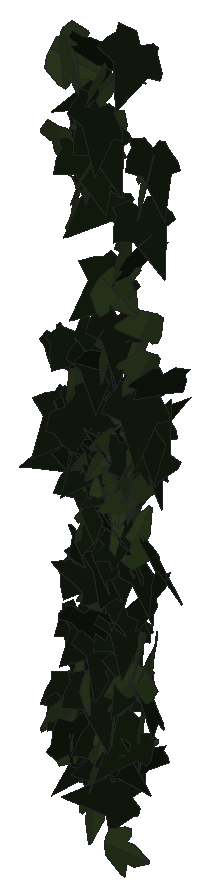
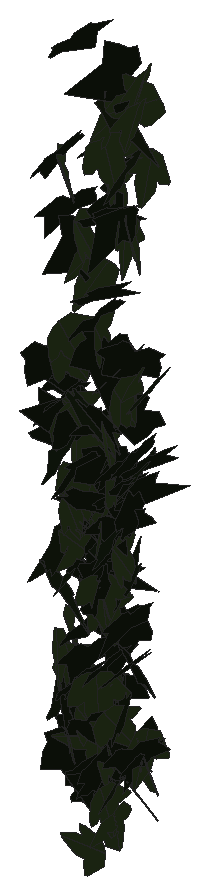
# SketchUp Ruby script. Lengths in inches.
U = 1.inch
M = Sketchup.active_model
def pt(a) = Geom::Point3d.new(a.map { |v| v * U })
def face(e, loops, mat)
  f = e.add_face(loops[0].map { |a| pt(a) })
  loops[1..].each { |l| e.add_face(l.map { |a| pt(a) }).erase! }
  f.material = f.back_material = mat if mat
  f
end
# faces: each face lists its corners as indices into pts; further lists are holes
def faces(e, pts, list, mat = nil) = list.each { |f| face(e, (f[0].is_a?(Array) ? f : [f]).map { |l| l.map { |i| pts[i] } }, mat) }
# xy, xz, yz: faces in a plane at the given z, y or x. An outline is a flat list of corners, or four numbers for a rectangle; further outlines are holes
def ring(l) = l.size == 4 ? [[l[0], l[1]], [l[2], l[1]], [l[2], l[3]], [l[0], l[3]]] : l.each_slice(2).to_a
def flat(e, list, mat, &to3) = list.each { |f| face(e, (f[0].is_a?(Array) ? f : [f]).map { |l| ring(l).map { |u, v| to3.(u, v) } }, mat) }
def xy(e, z, list, mat = nil) = flat(e, list, mat) { |x, y| [x, y, z] }
def xz(e, y, list, mat = nil) = flat(e, list, mat) { |x, z| [x, y, z] }
def yz(e, x, list, mat = nil) = flat(e, list, mat) { |y, z| [x, y, z] }
def lines(e, pts, list) = list.each { |a, b| e.add_line(pt(pts[a]), pt(pts[b])) }
# prism: a flat outline (further loops are holes) pulled along v
def prism(e, loops, v, mat = nil)
  f = face(e, loops, mat); d = Geom::Vector3d.new(v.map { |x| x * U })
  f.pushpull(f.normal.samedirection?(d) ? d.length : -d.length)
end
def box(e, o, s, mat = nil) = prism(e, [[o, [o[0] + s[0], o[1], o[2]], [o[0] + s[0], o[1] + s[1], o[2]], [o[0], o[1] + s[1], o[2]]]], [0, 0, s[2]], mat)
def at(x, y, z, deg = 0) = Geom::Transformation.translation(pt([x, y, z])) * Geom::Transformation.rotation(ORIGIN, Z_AXIS, deg.degrees)
def axes(o, x, y, z) = Geom::Transformation.new([*x, 0, *y, 0, *z, 0, *pt(o).to_a, 1])
def part(name) = M.definitions.add(name)
# library, detail: a bought-in or finely detailed component or shape, given as its bounding box
def library(name, o, s) = part(name).tap { |d| box(d.entities, o, s) }
def detail(e, o, s) = box(e.add_group.entities, o, s)
def put(e, d, t, mat = nil) = e.add_instance(d, t).tap { |i| i.material = mat if mat }
def group(e, t, mat = nil) = e.add_group.tap { |g| g.transformation = t; g.material = mat if mat }.entities
root = M.entities
M.materials.add("efeu1").color = [18, 25, 13]
M.materials.add("efeu2").color = [43, 57, 29]
c1 = part("ivyleaf_9")
p = [[1.54,2.16,1.25],[1.36,2.04,1.19],[-0.21,0.99,0.68],[-0.71,1.11,0.82],[-0.85,0.86,0.67],[-0.8,0.17,0.21],
  [-0.9,-0.01,0.1],[-0.67,-0.16,-0.02],[-0.08,-0.08,-0.05],[-0.03,-0.6,-0.4],[0.65,-0.88,-0.66],[0.83,-0.6,-0.49],
  [1.29,-0.42,-0.43],[1.8125,-0.07,-0.26],[1.21,0.44,0.15]]
faces(c1.entities,p,[[0,1,2,3,4,5,6,7,8,9,10,11,12,13,14]],"efeu1")
c2 = part("ivyleaf_10")
p = [[0,0.5,-0.03],[-0.0625,2.02,-0.43],[-0.19,2.01,-0.46],[-0.54,1.05,-0.29],[-0.52,0.625,-0.18],[-0.83,0.76,-0.28],
  [-1.16,0.64,-0.33],[-1.15,0.33,-0.24],[-0.77,-0.39,0.02],[-0.3,-0.51,0.16],[0.04,-0.48,0.23],[-0.02,2.01,-0.4375],
  [-0.06,2.01,-0.43],[0.04,-0.49,0.23],[0.67,-0.49,0.14],[1.38,0.36,-0.2],[1.375,0.51,-0.24],[0.81,0.65,-0.19],
  [0.62,0.59,-0.15],[0.6,1.09,-0.28],[0.5,1.23,-0.31]]
faces(c2.entities,p,[[0,1,2,3,4,5,6,7,8,9,10],[11,12,0,13,14,15,16,17,18,19,20]],"efeu2")
put(root,c1,axes([547.32,131.42,224.66],[-0.47868,-0.70634,0.46293],[-0.07674,-0.49354,-0.8324],[0.84104,-0.44705,0.18753]))
put(root,c1,axes([547.71,131.58,223.14],[-0.49322,-0.36938,0.71696],[-0.52746,-0.48802,-0.61429],[0.61013,-0.7205,0.04852]))
put(root,c1,axes([547.15,132.01,211.76],[-0.22016,-0.88269,-0.2571],[0.05857,0.25037,-0.90972],[0.9175,-0.22779,-0.00362]))
put(root,c1,axes([547.45,132.16,222.26],[-0.04191,-0.03531,0.93001],[-0.38732,-0.84584,-0.04957],[0.84625,-0.38888,0.02337]))
put(root,c2,axes([547.47,130.75,211.55],[-0.18429,-0.84828,-0.40002],[0.1268,0.38139,-0.86719],[0.92926,-0.22027,0.039]))
put(root,c1,axes([547.14,131.29,211.23],[0.26036,-0.7735,-0.32739],[-0.09812,0.3124,-0.81612],[0.83418,0.27816,0.00618]))
put(root,c1,axes([547.01,130.96,228.1875],[0.58686,-0.6803,-0.30129],[-0.06346,0.33656,-0.88357],[0.74132,0.56737,0.16287]))
put(root,c2,axes([547.39,131.55,241.125],[-0.02007,0.99355,0.08252],[0.00579,0.08265,-0.99372],[-0.99695,-0.01953,-0.00743]))
put(root,c2,axes([547.71,130.32,238.18],[-0.98634,0.09088,0.02629],[-0.02805,-0.01793,-0.99031],[-0.09035,-0.98653,0.02042]))
put(root,c2,axes([547.59,130.89,242.27],[-0.23804,0.98869,0.08205],[-0.01701,0.0803,-1.01694],[-0.99194,-0.23864,-0.00225]))
put(root,c2,axes([547.66,131.57,235.55],[0.54123,-0.82841,0.07096],[0.05419,-0.04934,-0.98937],[0.82967,0.54362,0.01833]))
put(root,c2,axes([547.33,130.66,209.71],[0.83861,-0.57924,-0.33432],[0.2838,-0.17731,1.0191],[-0.6056,-0.88521,0.01463]))
put(root,c1,axes([547.26,131.54,224.36],[0.3636,-0.84522,0.18301],[0.08963,-0.16063,-0.91993],[0.86015,0.37403,0.01849]))
put(root,c1,axes([547.47,131.55,215.46],[-0.46735,-0.24401,-0.71496],[0.74885,-0.03877,-0.47627],[0.09963,-0.85327,0.2261]))
put(root,c2,axes([547.24,130.92,241.41],[0.31548,0.25093,0.93435],[0.69363,0.62644,-0.40243],[-0.67443,0.76165,0.02317]))
put(root,c1,axes([547.54,131.38,225.12],[0.34402,-0.81704,-0.3168],[-0.126,0.29068,-0.88651],[0.8672,0.36636,-0.00313]))
put(root,c1,axes([547.64,131.59,217.67],[0.26274,-0.70515,-0.50734],[-0.07363,0.51005,-0.74705],[0.86557,0.25744,0.09045]))
put(root,c2,axes([547.63,131.04,210.85],[-0.20357,0.20119,-0.88456],[0.38608,-0.80114,-0.27107],[-0.82089,-0.42668,0.09188]))
put(root,c1,axes([547.73,132.27,212.72],[-0.0895,-0.19387,0.91513],[0.13572,-0.91228,-0.17999],[0.92554,0.11503,0.11488]))
put(root,c2,axes([548.24,132.12,212.84],[-0.40315,-0.58171,0.56523],[-0.04105,-0.61576,-0.663],[0.81006,-0.32072,0.24771]))
put(root,c2,axes([548.1,131.71,220.34],[0.27034,-0.74396,0.51626],[0.19524,-0.47821,-0.79138],[0.88424,0.33304,0.0169]))
put(root,c2,axes([548.3,131.02,235.13],[0.15158,-0.92217,-0.3501],[0.02552,0.35776,-0.93129],[0.98606,0.1325,0.07792]))
put(root,c1,axes([548.25,131.75,214.76],[-0.39192,-0.63578,0.60141],[-0.03798,-0.64598,-0.70765],[0.87433,-0.31305,0.23884]))
put(root,c1,axes([547.9,131.8,224.8],[0.28671,-0.85198,-0.28202],[0.00517,0.29762,-0.89387],[0.89743,0.27047,0.09525]))
put(root,c1,axes([548.9375,131.03,240.46],[-0.70581,0.71174,-0.00258],[-0.13908,-0.14148,-0.98254],[-0.69802,-0.69149,0.19838]))
put(root,c1,axes([548.15,131.79,222.04],[-0.3064,-0.87543,-0.31963],[0.13386,0.29163,-0.92707],[0.92229,-0.33316,0.02837]))
put(root,c2,axes([548.06,131.22,227.31],[-0.09751,-0.30544,0.97975],[0.5556,-0.84317,-0.20756],[0.86285,0.50841,0.24437]))
put(root,c1,axes([548.78,130.81,209.66],[-0.83384,0.27462,-0.12822],[0.11727,-0.05375,-0.87778],[-0.27947,-0.84193,0.01421]))
put(root,c1,axes([548.29,131.38,236.13],[0.91272,0.16773,-0.33496],[-0.34294,0.0191,-0.92489],[-0.15075,0.97206,0.07597]))
put(root,c1,axes([548.47,131.75,223.1],[-0.42551,-0.70439,0.44819],[-0.11444,-0.44909,-0.81444],[0.82701,-0.42456,0.1179]))
put(root,c1,axes([548.12,131.4,218.51],[0.62788,-0.5745,-0.46011],[0.38815,-0.25542,0.84858],[-0.62538,-0.73532,0.06473]))
put(root,c2,axes([548.41,131.29,227.4],[0.11453,-0.81074,0.55762],[0.24872,-0.5193,-0.80612],[0.95204,0.2332,0.14352]))
put(root,c1,axes([547.98,131.49,238],[0.5069,-0.83393,0.20261],[0.10523,-0.17314,-0.9759],[0.85171,0.51771,-0.00002]))
put(root,c2,axes([548.64,131.25,223.44],[0.07915,-0.92586,0.10516],[0.02453,-0.10343,-0.92911],[0.93149,0.0814,0.01553]))
put(root,c1,axes([548.45,129.94,210.08],[-0.17006,-0.19771,0.96973],[0.68393,0.68771,0.26015],[-0.71533,0.70452,0.0182]))
put(root,c1,axes([548.15,132.06,221.29],[0.52736,-0.78971,0.23886],[0.10385,-0.21769,-0.94901],[0.81848,0.53644,-0.03348]))
put(root,c2,axes([549.01,130.94,240.05],[0.01364,-0.0121,1.00923],[-0.41848,0.9184,0.01667],[-0.91845,-0.41864,0.00739]))
put(root,c2,axes([549.04,131.82,218.66],[-0.78887,-0.39575,0.18638],[-0.1283,-0.15811,-0.87876],[0.4182,-0.79502,0.08199]))
put(root,c1,axes([548.38,130.44,229.11],[-0.10535,-0.57039,-0.78902],[0.32065,0.72902,-0.56983],[0.91928,-0.31965,0.10833]))
put(root,c2,axes([548.9375,131.49,225.71],[0.37454,-0.85823,-0.17643],[-0.05543,0.16828,-0.93626],[0.87442,0.37828,0.01622]))
put(root,c1,axes([548.57,131.3125,223.78],[0.62831,-0.58568,-0.45673],[-0.32691,0.31909,-0.8589],[0.6669,0.7082,0.00927]))
put(root,c2,axes([549.03,131.46,238.83],[-0.48059,-0.84701,0.21226],[-0.02972,-0.22628,-0.97024],[0.87269,-0.47415,0.08385]))
put(root,c2,axes([548.78,131.22,207.66],[0.09175,0.92056,-0.34703],[-0.05828,-0.34284,-0.92485],[-0.98207,0.10635,0.02246]))
put(root,c1,axes([549.3,131.29,218.85],[-0.76483,-0.53418,0.18892],[0.16843,0.08868,0.93262],[-0.54099,0.78281,0.02326]))
put(root,c2,axes([548.99,131.58,208.7],[-0.13905,-0.85619,0.22979],[0.09011,-0.24505,-0.8585],[0.8819,-0.10996,0.12395]))
put(root,c1,axes([549.25,130.9375,224.1],[0.30233,0.76918,-0.4325],[-0.27731,-0.35121,-0.81844],[-0.83773,0.39385,0.11484]))
put(root,c1,axes([548.27,130.91,242.18],[0.90725,-0.10553,0.4551],[0.4522,-0.05131,-0.91337],[0.11734,1.0137,0.00114]))
put(root,c2,axes([549.16,131.29,221.875],[-0.52382,0.71468,0.32697],[-0.21558,0.24721,-0.88571],[-0.75578,-0.56585,0.02602]))
put(root,c2,axes([549.11,130.76,237.16],[0.25674,-0.95513,0.03323],[0.00963,-0.03182,-0.98904],[0.95566,0.25691,0.00104]))
put(root,c2,axes([549.33,131.71,213.93],[-0.84794,-0.54917,0.14085],[-0.11342,-0.08397,-1.0102],[0.55548,-0.85544,0.00874]))
put(root,c1,axes([548.54,129.75,226.08],[0.40363,-0.08687,-0.96647],[0.15011,1.03974,-0.03077],[0.95869,-0.12623,0.41173]))
put(root,c1,axes([549.16,130.04,216.57],[0.74863,0.51234,-0.44094],[-0.37747,-0.22895,-0.9069],[-0.56075,0.83812,0.02181]))
put(root,c1,axes([549.4,131.53,235.55],[-0.69557,-0.5992,0.35237],[-0.10079,-0.40628,-0.88983],[0.68778,-0.66552,0.22596]))
put(root,c1,axes([549.98,130.18,218.39],[-0.50022,0.24562,0.72164],[-0.6564,0.3001,-0.55713],[-0.38761,-0.82518,0.01218]))
put(root,c1,axes([548.74,131.23,209.19],[0.52091,-0.72414,0.12094],[0.05975,-0.10598,-0.89194],[0.73174,0.52415,-0.01326]))
put(root,c2,axes([549.44,131.1,217.41],[-0.20158,-0.8945,0.24019],[-0.03217,-0.2389,-0.9167],[0.92563,-0.2031,0.02044]))
put(root,c1,axes([549.47,131.91,226.71],[-0.89317,-0.12559,-0.3101],[0.30667,0.0461,-0.90196],[0.13376,-0.94435,-0.00279]))
put(root,c1,axes([549.08,131.43,214.79],[-0.08928,-0.92092,0.19135],[-0.00797,-0.19146,-0.92518],[0.94055,-0.08904,0.01032]))
put(root,c1,axes([549.97,130.45,211.05],[-0.80389,0.26072,0.29631],[-0.28211,0.09063,-0.84511],[-0.27602,-0.85196,0.00077]))
put(root,c1,axes([549.35,132.14,212.43],[-0.51011,-0.73714,-0.09526],[0.03853,0.08916,-0.89623],[0.74227,-0.51121,-0.01895]))
put(root,c1,axes([548.92,130.6,237.93],[-0.19068,-0.88096,-0.41769],[0.4461,0.29961,-0.83555],[0.86692,-0.34794,0.33808]))
put(root,c2,axes([549.07,131.54,218.32],[0.44504,-0.46695,0.62702],[0.48061,-0.40564,-0.64322],[0.61661,0.6532,0.0488]))
put(root,c1,axes([549.03,130.79,228.11],[0.05625,-0.89286,0.33367],[0.15148,-0.32163,-0.88618],[0.94106,0.10514,0.1227]))
put(root,c2,axes([549.35,130.35,213.43],[0.02992,0.83877,0.57828],[-0.02566,0.57896,-0.83844],[-1.01847,0.01005,0.03811]))
put(root,c1,axes([549.22,130.83,239.6],[0.04044,-0.98083,0.27735],[0.03894,-0.27588,-0.98131],[1.01855,0.04948,0.0265]))
put(root,c1,axes([548.97,132.04,218.32],[0.21479,-0.3171,0.87041],[0.44968,-0.74548,-0.38255],[0.80991,0.498,-0.01843]))
put(root,c1,axes([549.79,131.45,231.73],[-0.67035,-0.58293,0.40505],[-0.11603,-0.45964,-0.85352],[0.70029,-0.63416,0.24631]))
put(root,c1,axes([549.86,130.23,228.85],[0.27273,0.88988,-0.32008],[-0.11083,-0.30076,-0.93058],[-0.93917,0.2939,0.01687]))
put(root,c1,axes([549.81,131.62,209.28],[-0.26901,-0.33244,0.91473],[-0.45053,-0.79869,-0.42277],[0.86271,-0.52076,0.06445]))
put(root,c1,axes([550.14,132.17,222.54],[-0.84558,-0.26579,0.29779],[-0.25454,-0.17829,-0.8819],[0.30746,-0.87858,0.08887]))
put(root,c2,axes([549.62,130.74,210.28],[0.30491,-0.8303,0.57842],[0.28135,-0.51073,-0.88144],[0.97201,0.40829,0.07369]))
put(root,c1,axes([550.23,131.76,226.82],[-0.74832,0.55681,-0.11188],[0.0699,-0.09335,-0.93217],[-0.56362,-0.75085,0.03293]))
put(root,c1,axes([549.56,130.35,213.43],[-0.38609,-0.70133,-0.54457],[0.26402,0.47629,-0.80058],[0.84777,-0.46772,0.00131]))
put(root,c1,axes([549.16,131.48,219.75],[0.20568,-0.38388,0.87576],[0.5073,-0.71552,-0.43278],[0.81054,0.54524,0.04864]))
put(root,c1,axes([549.4,130.6875,238.91],[0.17907,-0.9602,-0.24181],[0.0848,0.2597,-0.96845],[0.98654,0.15197,0.12713]))
put(root,c1,axes([550.46,130.83,220.29],[-0.81708,0.37026,0.15557],[-0.14626,0.05411,-0.89699],[-0.37403,-0.82999,0.01092]))
put(root,c1,axes([549.65,131.8,215.57],[-0.01171,-0.81416,-0.42223],[0.016,0.42202,-0.8142],[0.917,-0.01776,0.00881]))
put(root,c1,axes([549.57,130.99,218.25],[-0.07467,-0.66203,0.67681],[0.20357,-0.67426,-0.63708],[0.92462,0.09498,0.19492]))
put(root,c2,axes([550.03,130.44,211.95],[0.70377,-0.55614,-0.18043],[-0.07491,0.19425,-0.89095],[0.57986,0.70008,0.10388]))
put(root,c1,axes([549.87,131.17,218.77],[-0.67841,-0.40843,-0.53311],[0.4378,0.30566,-0.7913],[0.50926,-0.80686,-0.02992]))
put(root,c1,axes([550,130.9,223.51],[0.57722,-0.78853,0.10991],[-0.05956,0.09261,0.9772],[-0.79392,-0.58024,0.0066]))
put(root,c2,axes([550.26,130.64,224.7],[0.28421,0.66329,-0.61443],[-0.44997,-0.45488,-0.69919],[-0.78423,0.50139,0.1785]))
put(root,c2,axes([549.96,131.25,222.64],[0.87545,0.50343,0.02185],[0.01774,0.01297,-1.00988],[-0.50359,0.87563,0.0024]))
put(root,c2,axes([549.93,130.67,229.5],[0.2614,-0.74865,0.54358],[0.36596,-0.43512,-0.77526],[0.84973,0.4177,0.16667]))
put(root,c1,axes([549.74,131.15,224.04],[0.29911,-0.58484,-0.6619],[0.01957,0.70304,-0.61235],[0.88305,0.18252,0.23777]))
put(root,c2,axes([550.14,131.49,212.2],[0.17575,-0.74951,0.53474],[0.15508,-0.51252,-0.76934],[0.90756,0.23272,0.02791]))
put(root,c1,axes([550.78,130.85,208.37],[-0.34485,-0.2154,0.89744],[-0.78713,-0.4316,-0.40605],[0.4819,-0.8591,-0.02102]))
put(root,c2,axes([550.73,131.17,222.1],[-0.61735,-0.50673,-0.6516],[-0.48202,-0.43923,0.79826],[-0.67009,0.78281,0.0261]))
put(root,c1,axes([550.16,130.8,230.27],[0.01811,-0.95532,0.01024],[-0.00789,-0.01039,-0.95546],[0.95535,0.01802,-0.00808]))
put(root,c2,axes([550.28,130.15,232.16],[0.31789,0.67844,0.62044],[0.09422,0.62899,-0.73606],[-0.91452,0.30063,0.13983]))
put(root,c1,axes([550.38,131.84,213.71],[-0.26912,-0.78092,0.38916],[-0.02686,-0.39964,-0.82053],[0.8721,-0.25329,0.09481]))
put(root,c2,axes([550.5,131.98,222.02],[0.10288,-0.85252,0.32302],[0.13225,-0.30768,-0.85414],[0.90202,0.14234,0.08838]))
put(root,c1,axes([550.26,131.34,216.29],[-0.02739,-0.93466,0.14007],[0.02004,-0.14068,-0.93475],[0.94488,-0.02411,0.02389]))
put(root,c2,axes([549.96,130.97,205.74],[-0.0496,0.00486,-0.90035],[0.8591,-0.2696,-0.04878],[-0.26945,-0.86047,0.0102]))
put(root,c2,axes([550.85,130.29,232.75],[-0.03346,0.04377,0.99083],[-0.41231,0.90105,-0.05373],[-0.90203,-0.41348,-0.0122]))
put(root,c2,axes([550.5625,131.02,219.59],[0.3139,0.61788,-0.69707],[0.21952,0.6658,0.68901],[0.90526,-0.3757,0.07463]))
put(root,c2,axes([550.07,130.32,210.65],[0.17341,-0.14546,-0.96569],[0.85175,0.50234,0.07728],[0.47775,-0.84279,0.21274]))
put(root,c2,axes([550.67,131,234.28],[0.35453,-0.82101,0.41816],[0.16123,-0.38585,-0.89427],[0.90715,0.38944,-0.00448]))
put(root,c1,axes([550.1,130.38,210.46],[0.07977,-0.0846,-0.88803],[0.79259,0.41585,0.03158],[0.40935,-0.78869,0.1119]))
put(root,c2,axes([550.86,131.84,229.875],[-0.28641,-0.80362,0.4711],[0.09897,-0.51633,-0.8206],[0.92626,-0.19332,0.23335]))
put(root,c2,axes([551.43,130.82,213.95],[-0.40886,-0.20733,0.77898],[-0.66565,-0.40581,-0.45738],[0.45465,-0.78058,0.03088]))
put(root,c1,axes([551.21,130.77,210.31],[0.07049,0.8965,-0.45168],[-0.079,-0.44643,-0.89842],[-1.00074,0.09839,0.03911]))
put(root,c2,axes([551.23,130.93,225.8],[-0.45056,-0.48996,0.68573],[-0.16217,-0.71264,-0.61574],[0.82704,-0.40666,0.25285]))
put(root,c1,axes([551.25,130.78,211.46],[-0.70486,-0.4847,0.14512],[-0.12381,-0.07607,-0.8554],[0.49058,-0.71561,-0.00737]))
put(root,c1,axes([550.58,131.46,218.84],[0.39257,-0.82947,0.10242],[0.0385,-0.09509,-0.91765],[0.83488,0.39441,-0.00584]))
put(root,c1,axes([550.88,131.87,212.95],[-0.42419,0.20028,-0.78486],[0.72829,-0.29349,-0.46851],[-0.35455,-0.84249,-0.02336]))
put(root,c2,axes([550.77,131.61,211.16],[0.49385,-0.61224,0.49872],[0.43187,-0.28304,-0.77513],[0.66109,0.64226,0.13381]))
put(root,c1,axes([551.05,130.23,233.11],[0.26033,0.54478,0.78932],[0.29039,0.73472,-0.60287],[-0.91405,0.38858,0.03327]))
put(root,c2,axes([551.26,130.4,224.01],[0.21042,-0.88213,-0.16879],[-0.03534,0.16509,-0.90687],[0.89744,0.21333,0.00386]))
put(root,c1,axes([551.0625,131.07,243.01],[-0.31745,-0.93045,0.24084],[-0.00011,-0.2536,-0.9799],[0.96111,-0.30736,0.07943]))
put(root,c2,axes([551.38,131.14,228.5],[-0.09761,-0.81256,0.56907],[0.0633,-0.57576,-0.81124],[0.98999,-0.0433,0.10798]))
put(root,c1,axes([551.94,131.05,217.85],[-0.64122,0.69311,0.21821],[-0.14879,0.15962,-0.94422],[-0.71125,-0.65825,0.0008]))
put(root,c2,axes([551.51,131.39,215.09],[0.24253,-0.82501,-0.4338],[-0.11986,0.41692,-0.85992],[0.92437,0.27052,0.00232]))
put(root,c2,axes([551.18,131.54,237.3125],[0.69988,-0.70381,0.33659],[0.23017,-0.24578,-0.99251],[0.74542,0.7367,-0.00956]))
put(root,c2,axes([551.41,131.18,225.25],[-0.17472,-0.69723,0.62679],[0.22243,-0.65021,-0.66127],[0.91078,0.02504,0.28174]))
put(root,c1,axes([551.16,130.65,225.14],[0.10303,0.10914,0.98023],[0.74106,0.6418,-0.14935],[-0.65084,0.74804,-0.01488]))
put(root,c2,axes([551.44,130.76,215.65],[0.56928,-0.68685,0.16456],[0.10083,-0.13016,-0.89209],[0.69906,0.57812,-0.00534]))
put(root,c1,axes([551.01,131.67,212.72],[0.17992,-0.66315,0.67163],[0.23842,-0.62962,-0.68554],[0.91324,0.29502,0.04666]))
put(root,c1,axes([551.02,131.8125,223.97],[0.34589,-0.79676,0.44921],[0.15084,-0.424,-0.86817],[0.90214,0.37638,-0.02708]))
put(root,c1,axes([551.22,131.07,235.5],[0.08512,-0.87813,-0.43831],[0.07292,0.44439,-0.87616],[0.97872,0.04326,0.1034]))
put(root,c1,axes([551.2,131.51,219.77],[0.77416,-0.49636,-0.12358],[-0.12216,0.03829,-0.91901],[0.49672,0.78303,-0.0334]))
put(root,c1,axes([551.27,131.74,238],[0.17979,-0.96531,-0.07932],[0.00251,0.08114,-0.98176],[0.96856,0.17897,0.01727]))
put(root,c1,axes([551.52,130.625,227.19],[-0.22147,-0.95738,-0.12023],[0.03653,0.11495,-0.98262],[0.96421,-0.22426,0.00961]))
put(root,c1,axes([551.76,130.38,224.11],[-0.66633,-0.14142,0.80916],[0.78729,0.18726,0.68106],[-0.23432,1.03134,-0.01271]))
put(root,c1,axes([551.59,131.21,226.11],[0.06733,-0.97691,0.01161],[0.00091,-0.01157,-0.97922],[0.97697,0.06734,0.00011]))
put(root,c1,axes([552.25,131.11,228.23],[-0.08367,0.64711,-0.67817],[-0.0239,-0.68212,-0.64793],[-0.93707,-0.04038,0.07708]))
